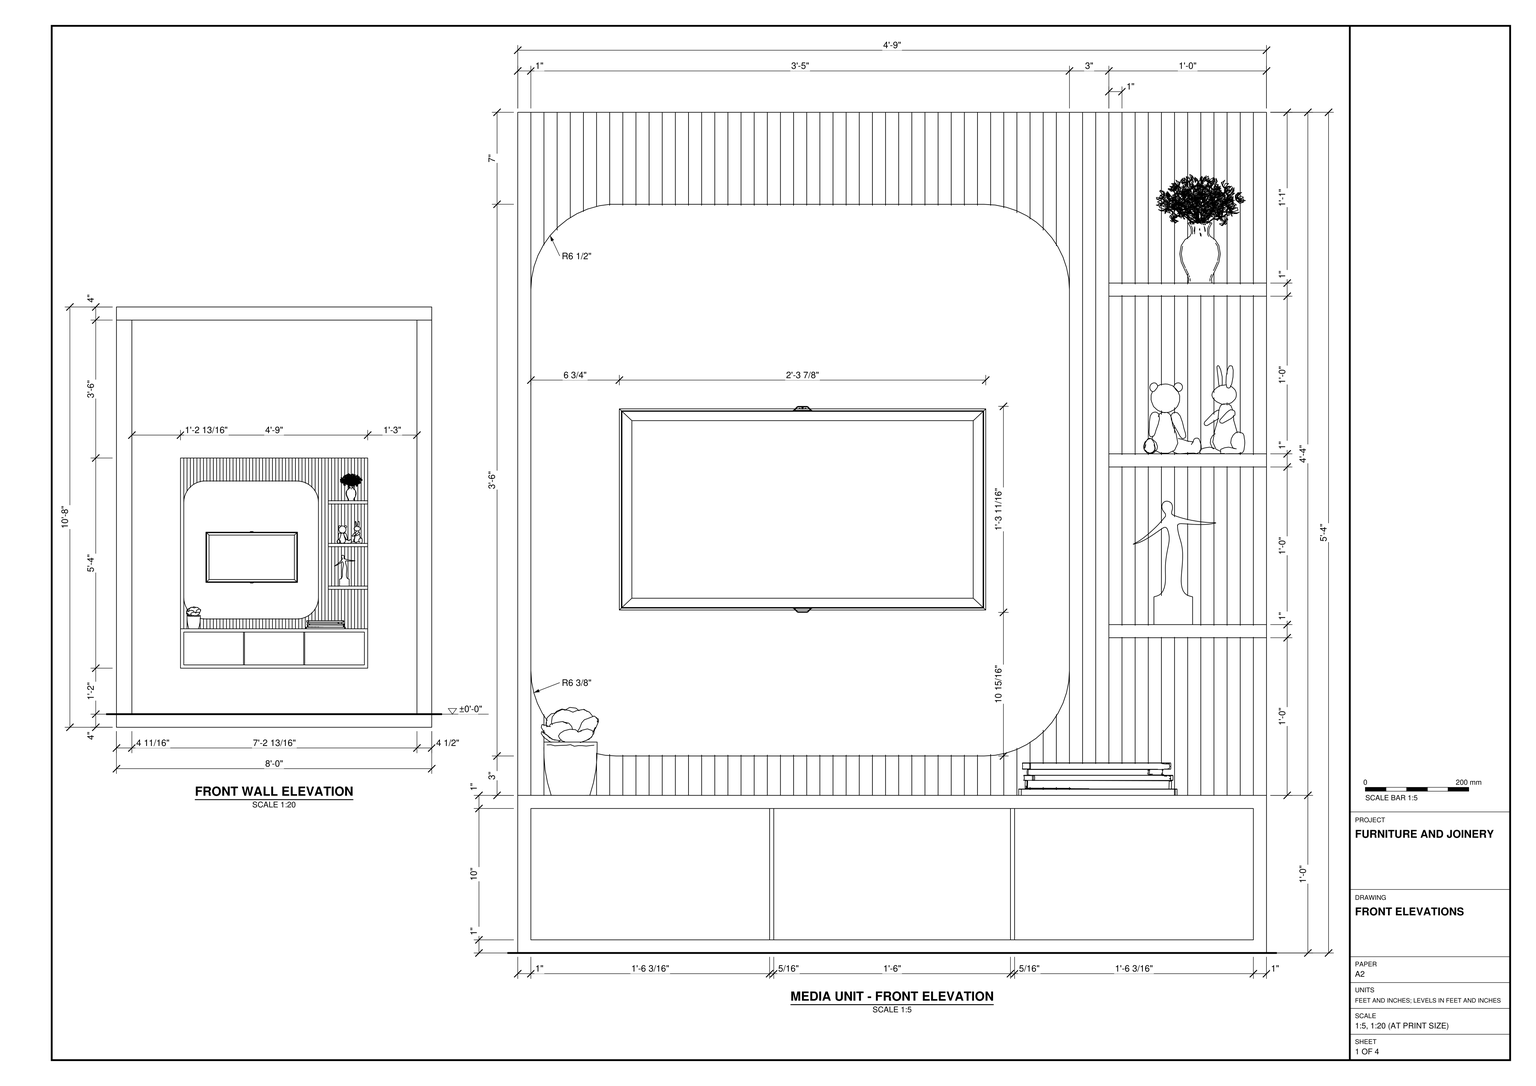
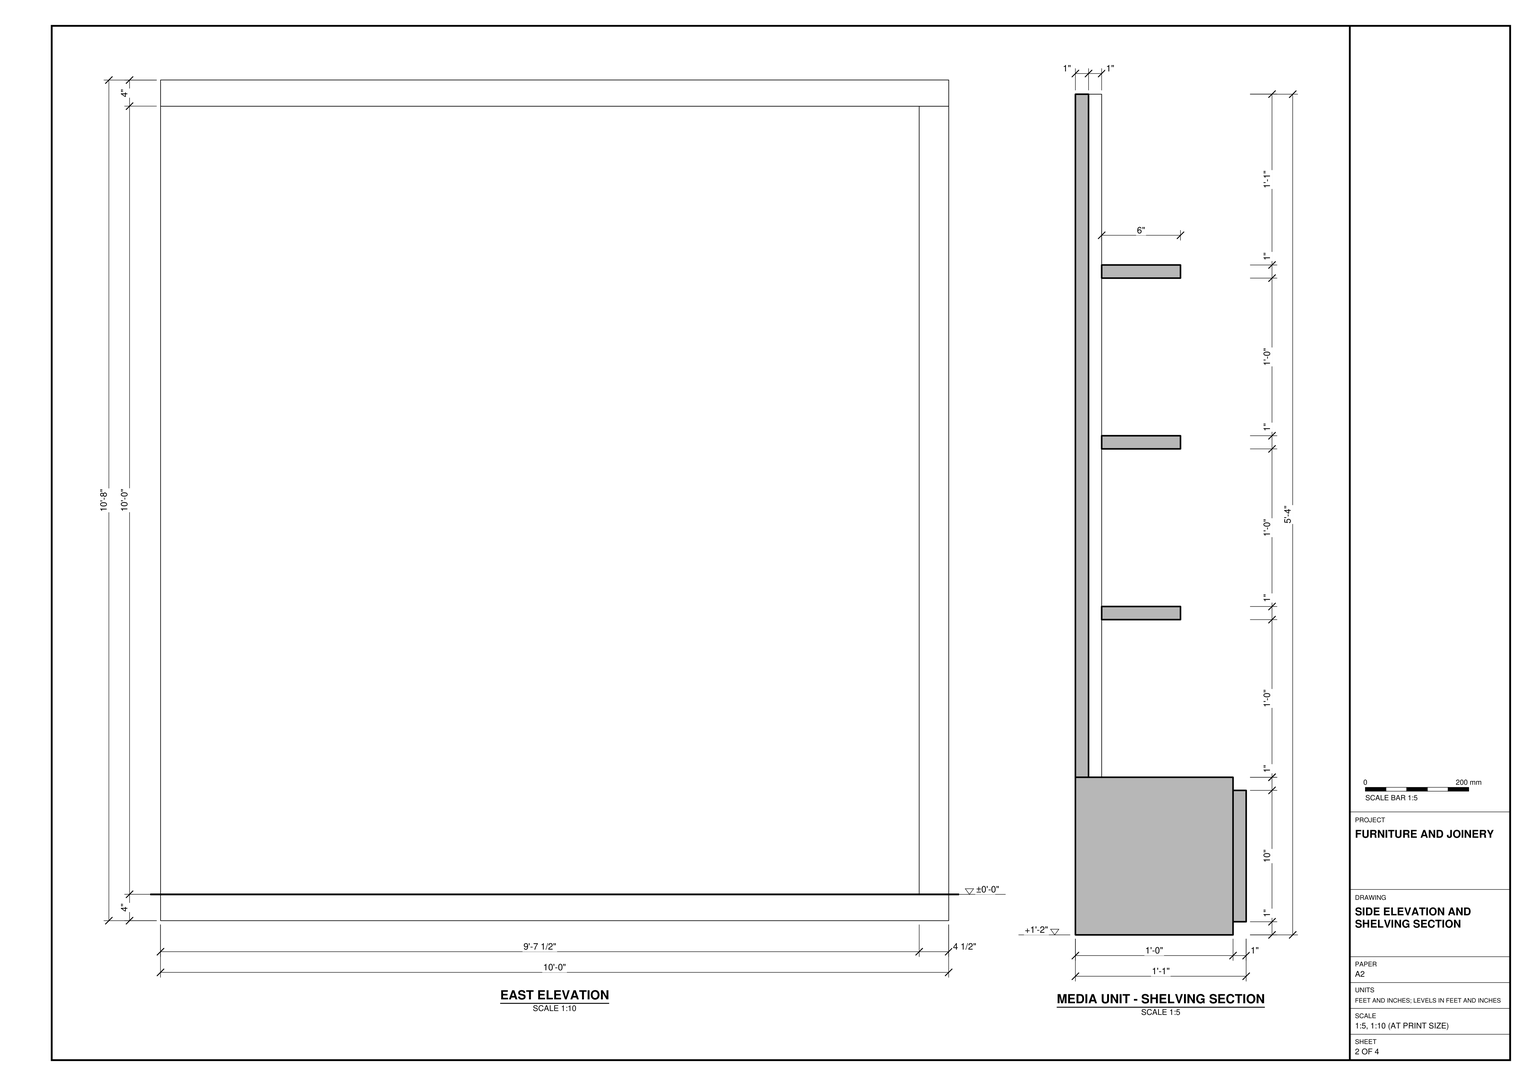
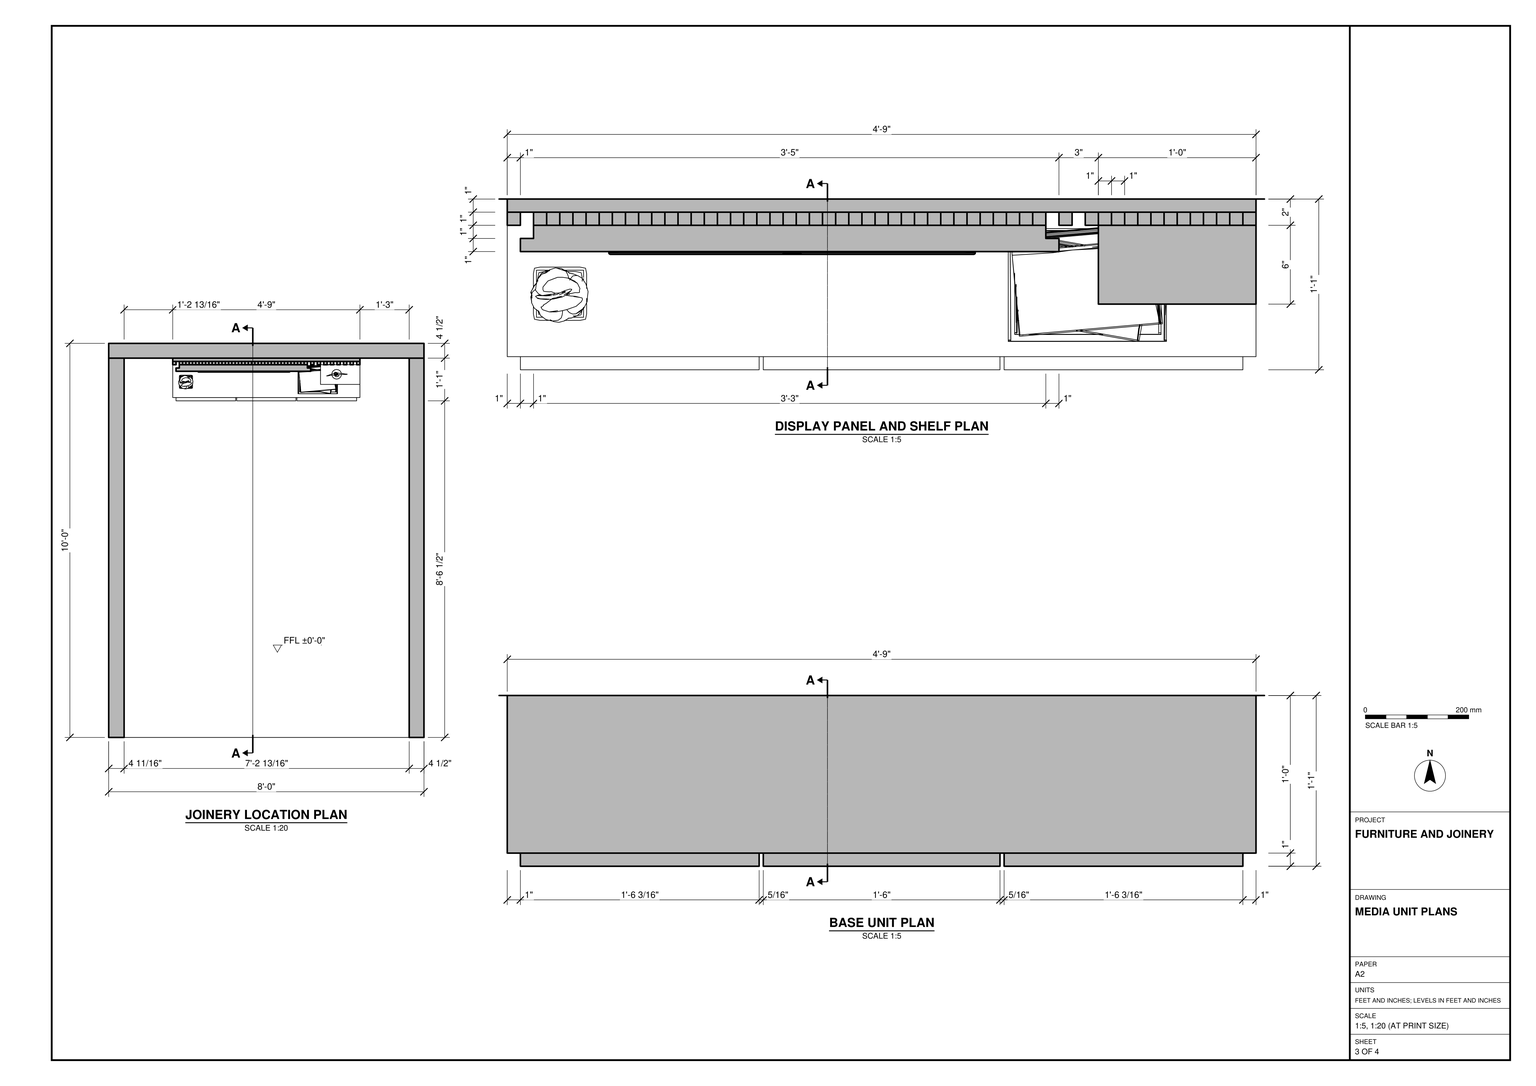
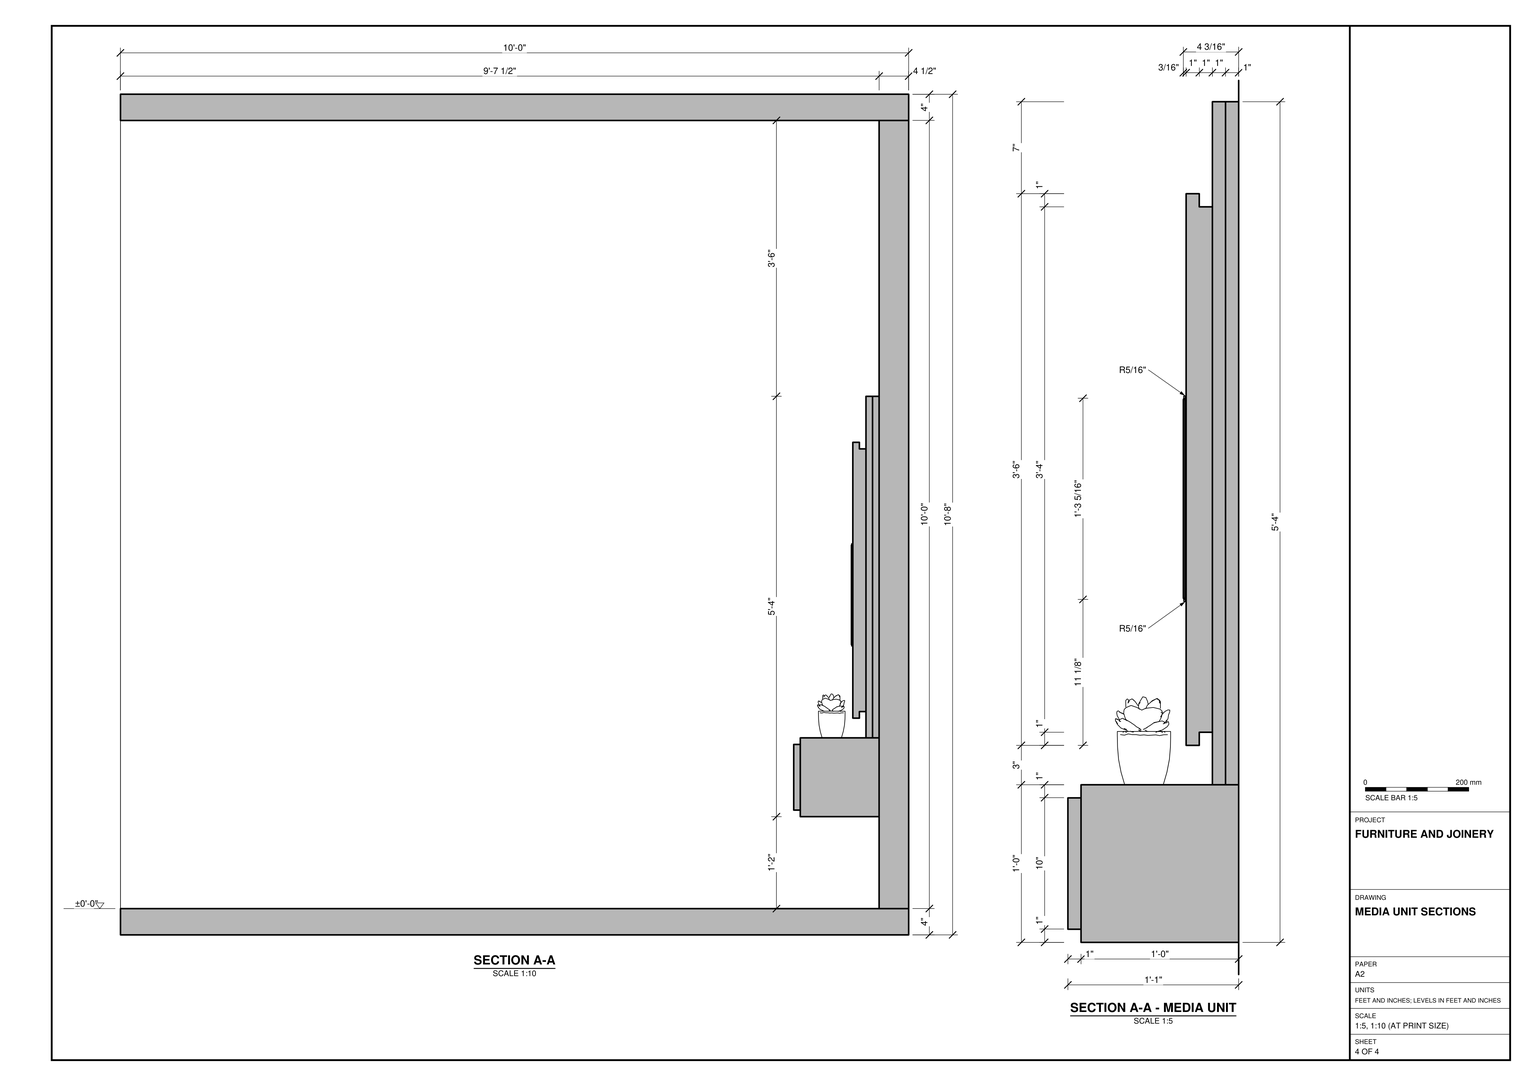
Build the wall-mounted media unit and its surrounding shell in SketchUp using task_files/diagram_01.pdf. Work in feet and inches. The overall model is 8'-0" wide, 10'-0" deep and 10'-8" high, with the finished floor at ±0'-0". Model the floor and overhead slabs, back wall and two side walls, leaving the front open as shown. Follow the individual wall thicknesses in the location plan.

Place the media unit against the back wall with its underside 1'-2" above the finished floor. The unit is 4'-9" wide and 5'-4" high. Form the floating base cabinet with three separate fronts and the narrow gaps shown in plan. Above it, model the vertical slatted backing, the projecting display panel with rounded corners, and the screen on the panel. Stack the shallow shelves to the right of the panel; use the shelving section to set their projection and spacing. Place the plant and books on the cabinet top and the display objects on their respective shelves. Decor and loose items may be any suitable library components, for example from 3D Warehouse.

Keep the walls, slabs and individual joinery pieces in separate groups or components, and use components for repeated parts. Save one SketchUp model as output_files/floating_media_unit_with_display_shelves.skp.

# SketchUp Ruby script. Lengths in inches.
U = 1.inch
M = Sketchup.active_model
def pt(a) = Geom::Point3d.new(a.map { |v| v * U })
def face(e, loops, mat)
  f = e.add_face(loops[0].map { |a| pt(a) })
  loops[1..].each { |l| e.add_face(l.map { |a| pt(a) }).erase! }
  f.material = f.back_material = mat if mat
  f
end
# faces: each face lists its corners as indices into pts; further lists are holes
def faces(e, pts, list, mat = nil) = list.each { |f| face(e, (f[0].is_a?(Array) ? f : [f]).map { |l| l.map { |i| pts[i] } }, mat) }
# xy, xz, yz: faces in a plane at the given z, y or x. An outline is a flat list of corners, or four numbers for a rectangle; further outlines are holes
def ring(l) = l.size == 4 ? [[l[0], l[1]], [l[2], l[1]], [l[2], l[3]], [l[0], l[3]]] : l.each_slice(2).to_a
def flat(e, list, mat, &to3) = list.each { |f| face(e, (f[0].is_a?(Array) ? f : [f]).map { |l| ring(l).map { |u, v| to3.(u, v) } }, mat) }
def xy(e, z, list, mat = nil) = flat(e, list, mat) { |x, y| [x, y, z] }
def xz(e, y, list, mat = nil) = flat(e, list, mat) { |x, z| [x, y, z] }
def yz(e, x, list, mat = nil) = flat(e, list, mat) { |y, z| [x, y, z] }
def lines(e, pts, list) = list.each { |a, b| e.add_line(pt(pts[a]), pt(pts[b])) }
# prism: a flat outline (further loops are holes) pulled along v
def prism(e, loops, v, mat = nil)
  f = face(e, loops, mat); d = Geom::Vector3d.new(v.map { |x| x * U })
  f.pushpull(f.normal.samedirection?(d) ? d.length : -d.length)
end
def box(e, o, s, mat = nil) = prism(e, [[o, [o[0] + s[0], o[1], o[2]], [o[0] + s[0], o[1] + s[1], o[2]], [o[0], o[1] + s[1], o[2]]]], [0, 0, s[2]], mat)
def at(x, y, z, deg = 0) = Geom::Transformation.translation(pt([x, y, z])) * Geom::Transformation.rotation(ORIGIN, Z_AXIS, deg.degrees)
def axes(o, x, y, z) = Geom::Transformation.new([*x, 0, *y, 0, *z, 0, *pt(o).to_a, 1])
def part(name) = M.definitions.add(name)
# library, detail: a bought-in or finely detailed component or shape, given as its bounding box
def library(name, o, s) = part(name).tap { |d| box(d.entities, o, s) }
def detail(e, o, s) = box(e.add_group.entities, o, s)
def put(e, d, t, mat = nil) = e.add_instance(d, t).tap { |i| i.material = mat if mat }
def group(e, t, mat = nil) = e.add_group.tap { |g| g.transformation = t; g.material = mat if mat }.entities
root = M.entities
M.materials.add("Ceramic Sand 8.13cm").color = [255, 255, 255]
M.materials.add("Ecorel - epc61025 33.57cm").color = [255, 255, 255]
M.materials.add("Emissive").color = [255, 201, 138]
M.materials.add("Wood Teak 33-35 100cm").color = [135, 81, 33]
c1 = part("Display shelf")
box(c1.entities,[0,-6,0],[12,6,1],"Wood Teak 33-35 100cm")
c2 = part("Group12\#1")
p = [[0,0,0],[0,0,-0.93],[-0.38,0,-0.93],[2.49,-0.52,0],[-2.49,-0.52,0],[2.49,0.52,0],
  [2.49,0,0],[-2.49,0.52,0],[0.38,0,-0.93],[-2.49,0,0],[0,0,-1.51]]
lines(c2.entities,p,[[0,1],[1,2],[3,4],[5,6],[7,5],[1,8],[9,0],[0,6],[8,10],[4,9],[6,3],[2,10],
  [9,7]])
c3 = part("Rectangle Light")
put(c3.entities,c2,at(0,0,0))
c4 = part("Group14\#1")
p = [[0,0,0],[0,0,-1.01],[-0.38,0,-1.01],[2.5,-0.77,0],[-2.5,-0.77,0],[2.5,0.77,0],
  [2.5,0,0],[-2.5,0.77,0],[0.38,0,-1.01],[-2.5,0,0],[0,0,-1.64]]
lines(c4.entities,p,[[0,1],[1,2],[3,4],[5,6],[7,5],[1,8],[9,0],[0,6],[8,10],[4,9],[6,3],[2,10],
  [9,7]])
c5 = part("Rectangle Light\#1")
put(c5.entities,c4,at(0,0,0))
c6 = part("Group16\#1")
p = [[0,0,0],[0,0,-1.12],[-0.38,0,-1.12],[2.51,-1.11,0],[-2.51,-1.11,0],[2.51,1.11,0],
  [2.51,0,0],[-2.51,1.11,0],[0.38,0,-1.12],[-2.51,0,0],[0,0,-1.81]]
lines(c6.entities,p,[[0,1],[1,2],[3,4],[5,6],[7,5],[1,8],[9,0],[0,6],[8,10],[4,9],[6,3],[2,10],
  [9,7]])
c7 = part("Rectangle Light\#2")
put(c7.entities,c6,at(0,0,0))
c8 = part("Group18\#1")
p = [[0,0,0],[0,0,-9.11],[-4.38,0,-9.11],[28.5,-1,0],[-28.5,-1,0],[28.5,1,0],
  [28.5,0,0],[-28.5,1,0],[4.38,0,-9.11],[-28.5,0,0],[0,0,-14.75]]
lines(c8.entities,p,[[0,1],[1,2],[3,4],[5,6],[7,5],[1,8],[9,0],[0,6],[8,10],[4,9],[6,3],[2,10],
  [9,7]])
c9 = part("Rectangle Light\#3")
put(c9.entities,c8,at(0,0,0))
c10 = library("Television screen",[0,1.41,1.14],[35.92,0.28,20.21])
c11 = library("Vase Flowers 26-02",[-5.76,-5.9,0],[11.73,12.02,14.27])
c12 = library("Decorative Figures 02 65-28",[-3.68,-1.82,0],[7.71,3.84,6.72])
c13 = library("Sculpture 108-23",[-12.84,-6.01,0],[25.68,12.02,38.36])
c14 = library("Potted Plant 50-24",[-2.18,-2.1,0],[4.36,4.2,6.7])
c15 = library("Books 193 003",[-6.07,-4.15,0],[12.06,9.04,2.47])
c16 = part("Group\#1")
box(c16.entities,[0,0,0],[96,120,4])
c17 = part("Vertical wood slat")
box(c17.entities,[0,-1,0],[1,1,52],"Wood Teak 33-35 100cm")
put(root,c1,at(64.5,113.5,68),"Wood Teak 33-35 100cm")
put(root,c1,at(64.5,113.5,55))
put(root,c1,at(64.5,113.5,42))
put(root,c3,axes([69.99,112.98,67.99],[1,0,0],[0,-1,0],[0,0,1]))
put(root,c5,axes([70,112.73,54.99],[1,0,0],[0,-1,0],[0,0,1]))
put(root,c7,axes([70.01,112.39,41.99],[1,0,0],[0,-1,0],[0,0,1]))
put(root,c9,axes([48,114.5,17.99],[1,0,0],[0,-1,0],[0,0,0.11]))
put(root,c10,axes([27.23,110.19,43.04],[0.77637,0,0],[0,0.77637,0],[0,0,0.77637]))
put(root,c11,axes([71.44,110.92,69],[0.58,0,0],[0,0.58,0],[0,0,0.58]))
put(root,c12,at(70.82,109.62,56))
put(root,c13,axes([69.5,110.6,43],[0.245,0,0],[0,0.245,0],[0,0,0.245]))
put(root,c14,at(23.47,108.22,30))
put(root,c15,at(63.7,108.8,30))
put(root,c16,at(0,0,0))
g1 = group(root,at(0,115.5,4))
box(g1,[0,0,0],[96,4.5,120],"Ceramic Sand 8.13cm")
g2 = group(root,at(19.5,103.5,18),"Wood Teak 33-35 100cm")
xy(g2,0,[[0,0,57,12]],"Wood Teak 33-35 100cm")
xy(g2,12,[[0,0,57,12]],"Wood Teak 33-35 100cm")
xz(g2,0,[[[0,0,57,12],[1,1,56,11]],[1,1,56,11]],"Wood Teak 33-35 100cm")
xz(g2,12,[[0,0,57,12]],"Wood Teak 33-35 100cm")
yz(g2,0,[[0,0,12,12]],"Wood Teak 33-35 100cm")
yz(g2,57,[[0,0,12,12]],"Wood Teak 33-35 100cm")
g3 = group(root,at(20.5,102.5,19))
xy(g3,0,[[0,0,18.18,1],[18.49,0,36.51,1],[36.82,0,55,1]],"Ecorel - epc61025 33.57cm")
xy(g3,10,[[0,0,18.18,1],[18.49,0,36.51,1],[36.82,0,55,1]],"Ecorel - epc61025 33.57cm")
xz(g3,0,[[0,0,18.18,10],[18.49,0,36.51,10],[36.82,0,55,10]],"Ecorel - epc61025 33.57cm")
xz(g3,1,[[0,0,18.18,10],[18.49,0,36.51,10],[36.82,0,55,10]])
yz(g3,0,[[0,0,1,10]],"Ecorel - epc61025 33.57cm")
yz(g3,18.18,[[0,0,1,10]])
yz(g3,18.49,[[0,0,1,10]])
yz(g3,36.51,[[0,0,1,10]])
yz(g3,36.82,[[0,0,1,10]])
yz(g3,55,[[0,0,1,10]],"Ecorel - epc61025 33.57cm")
g4 = group(root,at(19.5,114.5,30),"Wood Teak 33-35 100cm")
xy(g4,0,[[0,0,57,1]],"Wood Teak 33-35 100cm")
xy(g4,52,[[0,0,57,1]],"Wood Teak 33-35 100cm")
xz(g4,0,[[0,0,55,52],[55,0,56,52]],"Wood Teak 33-35 100cm")
xz(g4,1,[[0,0,57,52]],"Wood Teak 33-35 100cm")
yz(g4,0,[[0,0,1,52]],"Wood Teak 33-35 100cm")
yz(g4,57,[[0,0,1,52]],"Wood Teak 33-35 100cm")
put(g4,c17,at(56,0,0))
put(g4,c17,at(54,0,0))
put(g4,c17,at(52,0,0))
put(g4,c17,at(50,0,0))
put(g4,c17,at(48,0,0))
put(g4,c17,at(46,0,0))
put(g4,c17,at(44,0,0))
put(g4,c17,at(42,0,0))
put(g4,c17,at(40,0,0))
put(g4,c17,at(38,0,0))
put(g4,c17,at(36,0,0))
put(g4,c17,at(34,0,0))
put(g4,c17,at(32,0,0))
put(g4,c17,at(30,0,0))
put(g4,c17,at(28,0,0))
put(g4,c17,at(26,0,0))
put(g4,c17,at(24,0,0))
put(g4,c17,at(22,0,0))
put(g4,c17,at(20,0,0))
put(g4,c17,at(18,0,0))
put(g4,c17,at(16,0,0))
put(g4,c17,at(14,0,0))
put(g4,c17,at(12,0,0))
put(g4,c17,at(10,0,0))
put(g4,c17,at(8,0,0))
put(g4,c17,at(6,0,0))
put(g4,c17,at(4,0,0))
put(g4,c17,at(2,0,0))
put(g4,c17,at(0,0,0))
g5 = group(root,at(20.5,111.5,33))
xy(g5,0,[[6.502,0,34.498,1]],"Ecorel - epc61025 33.57cm")
xy(g5,1,[[6.502,1,34.498,2]],"Emissive")
xy(g5,41,[[6.125,1,34.498,2]],"Emissive")
xy(g5,42,[[6.058,0,34.498,1]],"Ecorel - epc61025 33.57cm")
xz(g5,0,[[6.502,0,34.498,0,35.346,0.056,36.181,0.222,36.986,0.495,37.749,0.871,38.456,1.344,39.096,1.904,39.656,2.544,40.129,3.251,40.505,4.014,40.778,4.819,40.944,5.654,41,6.502,41,35.498,40.944,36.346,40.778,37.181,40.505,37.986,40.129,38.749,39.656,39.456,39.096,40.096,38.456,40.656,37.749,41.129,36.986,41.505,36.181,41.778,35.346,41.944,34.498,42,6.058,42,5.194,41.883,4.338,41.646,3.522,41.293,2.761,40.832,2.071,40.272,1.463,39.624,0.95,38.898,0.54,38.109,0.242,37.271,0.061,36.401,0,35.514,0,6.502,0.056,5.654,0.222,4.819,0.495,4.014,0.871,3.251,1.344,2.544,1.904,1.904,2.544,1.344,3.251,0.871,4.014,0.495,4.819,0.222,5.654,0.056],[6.058,42,6.964,42,6.075,42.002]],"Ecorel - epc61025 33.57cm")
xz(g5,1,[[[6.502,0,5.654,0.056,4.819,0.222,4.014,0.495,3.251,0.871,2.544,1.344,1.904,1.904,1.344,2.544,0.871,3.251,0.495,4.014,0.222,4.819,0.056,5.654,0,6.502,0,35.514,0.061,36.401,0.242,37.271,0.54,38.109,0.95,38.898,1.463,39.624,2.071,40.272,2.761,40.832,3.522,41.293,4.338,41.646,5.194,41.883,6.058,42,34.498,42,35.346,41.944,36.181,41.778,36.986,41.505,37.749,41.129,38.456,40.656,39.096,40.096,39.656,39.456,40.129,38.749,40.505,37.986,40.778,37.181,40.944,36.346,41,35.498,41,6.502,40.944,5.654,40.778,4.819,40.505,4.014,40.129,3.251,39.656,2.544,39.096,1.904,38.456,1.344,37.749,0.871,36.986,0.495,36.181,0.222,35.346,0.056,34.498,0],[6.502,1,34.498,1,35.216,1.047,35.922,1.1875,36.603,1.419,37.249,1.737,37.847,2.137,38.388,2.612,38.863,3.153,39.263,3.751,39.581,4.397,39.8125,5.078,39.953,5.784,40,6.502,40,35.498,39.953,36.216,39.8125,36.922,39.581,37.603,39.263,38.249,38.863,38.847,38.388,39.388,37.847,39.863,37.249,40.263,36.603,40.581,35.922,40.8125,35.216,40.953,34.498,41,6.125,41,5.396,40.902,4.671,40.7,3.981,40.402,3.338,40.013,2.754,39.539,2.24,38.99,1.806,38.376,1.459,37.709,1.207,37,1.054,36.264,1,35.48,1,6.502,1.047,5.784,1.1875,5.078,1.419,4.397,1.737,3.751,2.137,3.153,2.612,2.612,3.153,2.137,3.751,1.737,4.397,1.419,5.078,1.1875,5.784,1.047]]],"Ecorel - epc61025 33.57cm")
xz(g5,2,[[6.502,1,5.784,1.047,5.078,1.1875,4.397,1.419,3.751,1.737,3.153,2.137,2.612,2.612,2.137,3.153,1.737,3.751,1.419,4.397,1.1875,5.078,1.047,5.784,1,6.502,1,35.48,1.054,36.264,1.207,37,1.459,37.709,1.806,38.376,2.24,38.99,2.754,39.539,3.338,40.013,3.981,40.402,4.671,40.7,5.396,40.902,6.125,41,34.498,41,35.216,40.953,35.922,40.8125,36.603,40.581,37.249,40.263,37.847,39.863,38.388,39.388,38.863,38.847,39.263,38.249,39.581,37.603,39.8125,36.922,39.953,36.216,40,35.498,40,6.502,39.953,5.784,39.8125,5.078,39.581,4.397,39.263,3.751,38.863,3.153,38.388,2.612,37.847,2.137,37.249,1.737,36.603,1.419,35.922,1.1875,35.216,1.047,34.498,1]],"Ecorel - epc61025 33.57cm")
yz(g5,0,[[0,6.502,1,35.514]],"Ecorel - epc61025 33.57cm")
yz(g5,1,[[1,6.502,2,35.48]],"Emissive")
yz(g5,40,[[1,6.502,2,35.498]],"Emissive")
yz(g5,41,[[0,6.502,1,35.498]],"Ecorel - epc61025 33.57cm")
p = [[6.502,0,0],[5.654,0,0.056],[5.654,1,0.056],[6.502,1,0],[35.346,0,0.056],[34.498,0,0],
  [34.498,1,0],[35.346,1,0.056],[4.819,0,0.222],[4.819,1,0.222],[36.181,0,0.222],[36.181,1,0.222],
  [4.014,0,0.495],[4.014,1,0.495],[36.986,0,0.495],[36.986,1,0.495],[3.251,0,0.871],[3.251,1,0.871],
  [37.749,0,0.871],[37.749,1,0.871],[2.544,0,1.344],[2.544,1,1.344],[38.456,0,1.344],[38.456,1,1.344],
  [5.784,1,1.047],[5.078,1,1.1875],[5.078,2,1.1875],[5.784,2,1.047],[6.502,1,1],[6.502,2,1],
  [35.216,1,1.047],[34.498,1,1],[34.498,2,1],[35.216,2,1.047],[35.922,1,1.1875],[35.922,2,1.1875],
  [4.397,1,1.419],[4.397,2,1.419],[36.603,1,1.419],[36.603,2,1.419],[1.904,0,1.904],[1.904,1,1.904],
  [39.096,0,1.904],[39.096,1,1.904],[3.751,1,1.737],[3.751,2,1.737],[37.249,1,1.737],[37.249,2,1.737],
  [3.153,1,2.137],[3.153,2,2.137],[37.847,1,2.137],[37.847,2,2.137],[1.344,0,2.544],[1.344,1,2.544],
  [39.656,0,2.544],[39.656,1,2.544],[2.612,1,2.612],[2.612,2,2.612],[38.388,1,2.612],[38.388,2,2.612],
  [0.871,0,3.251],[0.871,1,3.251],[40.129,0,3.251],[40.129,1,3.251],[2.137,1,3.153],[2.137,2,3.153],
  [38.863,1,3.153],[38.863,2,3.153],[1.737,1,3.751],[1.737,2,3.751],[39.263,1,3.751],[39.263,2,3.751],
  [0.495,0,4.014],[0.495,1,4.014],[40.505,0,4.014],[40.505,1,4.014],[1.419,1,4.397],[1.419,2,4.397],
  [39.581,1,4.397],[39.581,2,4.397],[0.222,0,4.819],[0.222,1,4.819],[40.778,0,4.819],[40.778,1,4.819],
  [1.1875,1,5.078],[1.1875,2,5.078],[39.8125,1,5.078],[39.8125,2,5.078],[0.056,0,5.654],[0.056,1,5.654],
  [40.944,0,5.654],[40.944,1,5.654],[1.047,1,5.784],[1.047,2,5.784],[39.953,1,5.784],[39.953,2,5.784],
  [0,0,6.502],[0,1,6.502],[41,0,6.502],[41,1,6.502],[1,1,6.502],[1,2,6.502],
  [40,1,6.502],[40,2,6.502],[0,0,35.514],[0.061,0,36.401],[0.061,1,36.401],[0,1,35.514],
  [40.944,0,36.346],[41,0,35.498],[41,1,35.498],[40.944,1,36.346],[1,1,35.48],[1.054,1,36.264],
  [1.054,2,36.264],[1,2,35.48],[39.953,1,36.216],[40,1,35.498],[40,2,35.498],[39.953,2,36.216],
  [39.8125,1,36.922],[39.8125,2,36.922],[40.778,0,37.181],[40.778,1,37.181],[1.207,1,37],[1.207,2,37],
  [0.242,0,37.271],[0.242,1,37.271],[39.581,1,37.603],[39.581,2,37.603],[1.459,1,37.709],[1.459,2,37.709],
  [40.505,0,37.986],[40.505,1,37.986],[0.54,0,38.109],[0.54,1,38.109],[39.263,1,38.249],[39.263,2,38.249],
  [1.806,1,38.376],[1.806,2,38.376],[40.129,0,38.749],[40.129,1,38.749],[0.95,0,38.898],[0.95,1,38.898],
  [38.863,1,38.847],[38.863,2,38.847],[2.24,1,38.99],[2.24,2,38.99],[39.656,0,39.456],[39.656,1,39.456],
  [38.388,1,39.388],[38.388,2,39.388],[1.463,0,39.624],[1.463,1,39.624],[2.754,1,39.539],[2.754,2,39.539],
  [37.847,1,39.863],[37.847,2,39.863],[39.096,0,40.096],[39.096,1,40.096],[3.338,1,40.013],[3.338,2,40.013],
  [2.071,0,40.272],[2.071,1,40.272],[37.249,1,40.263],[37.249,2,40.263],[3.981,1,40.402],[3.981,2,40.402],
  [38.456,0,40.656],[38.456,1,40.656],[2.761,0,40.832],[2.761,1,40.832],[36.603,1,40.581],[36.603,2,40.581],
  [4.671,1,40.7],[4.671,2,40.7],[35.922,1,40.8125],[35.922,2,40.8125],[37.749,0,41.129],[37.749,1,41.129],
  [5.396,1,40.902],[5.396,2,40.902],[3.522,0,41.293],[3.522,1,41.293],[35.216,1,40.953],[35.216,2,40.953],
  [6.125,1,41],[6.125,2,41],[34.498,1,41],[34.498,2,41],[36.986,0,41.505],[36.986,1,41.505],
  [4.338,0,41.646],[4.338,1,41.646],[36.181,0,41.778],[36.181,1,41.778],[5.194,0,41.883],[5.194,1,41.883],
  [35.346,0,41.944],[35.346,1,41.944],[6.058,0,42],[6.058,1,42],[34.498,0,42],[34.498,1,42]]
faces(g5,p,[[0,1,2,3],[4,5,6,7],[1,8,9,2],[10,4,7,11],[8,12,13,9],[14,10,11,15],[12,16,17,13],[18,14,15,19],
  [16,20,21,17],[22,18,19,23],[20,40,41,21],[42,22,23,43],[40,52,53,41],[54,42,43,55],[52,60,61,53],[62,54,55,63],
  [60,72,73,61],[74,62,63,75],[72,80,81,73],[82,74,75,83],[80,88,89,81],[90,82,83,91],[88,96,97,89],[98,90,91,99],
  [104,105,106,107],[108,109,110,111],[122,108,111,123],[105,126,127,106],[132,122,123,133],[126,134,135,127],[140,132,133,141],[134,142,143,135],
  [148,140,141,149],[142,152,153,143],[158,148,149,159],[152,162,163,153],[168,158,159,169],[162,170,171,163],[178,168,169,179],[170,182,183,171],
  [190,178,179,191],[182,192,193,183],[194,190,191,195],[192,196,197,193],[198,194,195,199],[196,200,201,197],[202,198,199,203]],"Ecorel - epc61025 33.57cm")
faces(g5,p,[[24,25,26,27],[28,24,27,29],[30,31,32,33],[34,30,33,35],[25,36,37,26],[38,34,35,39],[36,44,45,37],[46,38,39,47],
  [44,48,49,45],[50,46,47,51],[48,56,57,49],[58,50,51,59],[56,64,65,57],[66,58,59,67],[64,68,69,65],[70,66,67,71],
  [68,76,77,69],[78,70,71,79],[76,84,85,77],[86,78,79,87],[84,92,93,85],[94,86,87,95],[92,100,101,93],[102,94,95,103],
  [112,113,114,115],[116,117,118,119],[120,116,119,121],[113,124,125,114],[128,120,121,129],[124,130,131,125],[136,128,129,137],[130,138,139,131],
  [144,136,137,145],[138,146,147,139],[150,144,145,151],[146,154,155,147],[156,150,151,157],[154,160,161,155],[164,156,157,165],[160,166,167,161],
  [172,164,165,173],[166,174,175,167],[176,172,173,177],[174,180,181,175],[184,176,177,185],[180,186,187,181],[188,184,185,189]],"Emissive")
g6 = group(root,at(91.5,0,4))
box(g6,[0,0,0],[4.5,115.5,120],"Ceramic Sand 8.13cm")
g7 = group(root,at(0,0,4))
box(g7,[0,0,0],[4.69,115.5,120],"Ceramic Sand 8.13cm")
put(root,c16,at(0,0,124))
